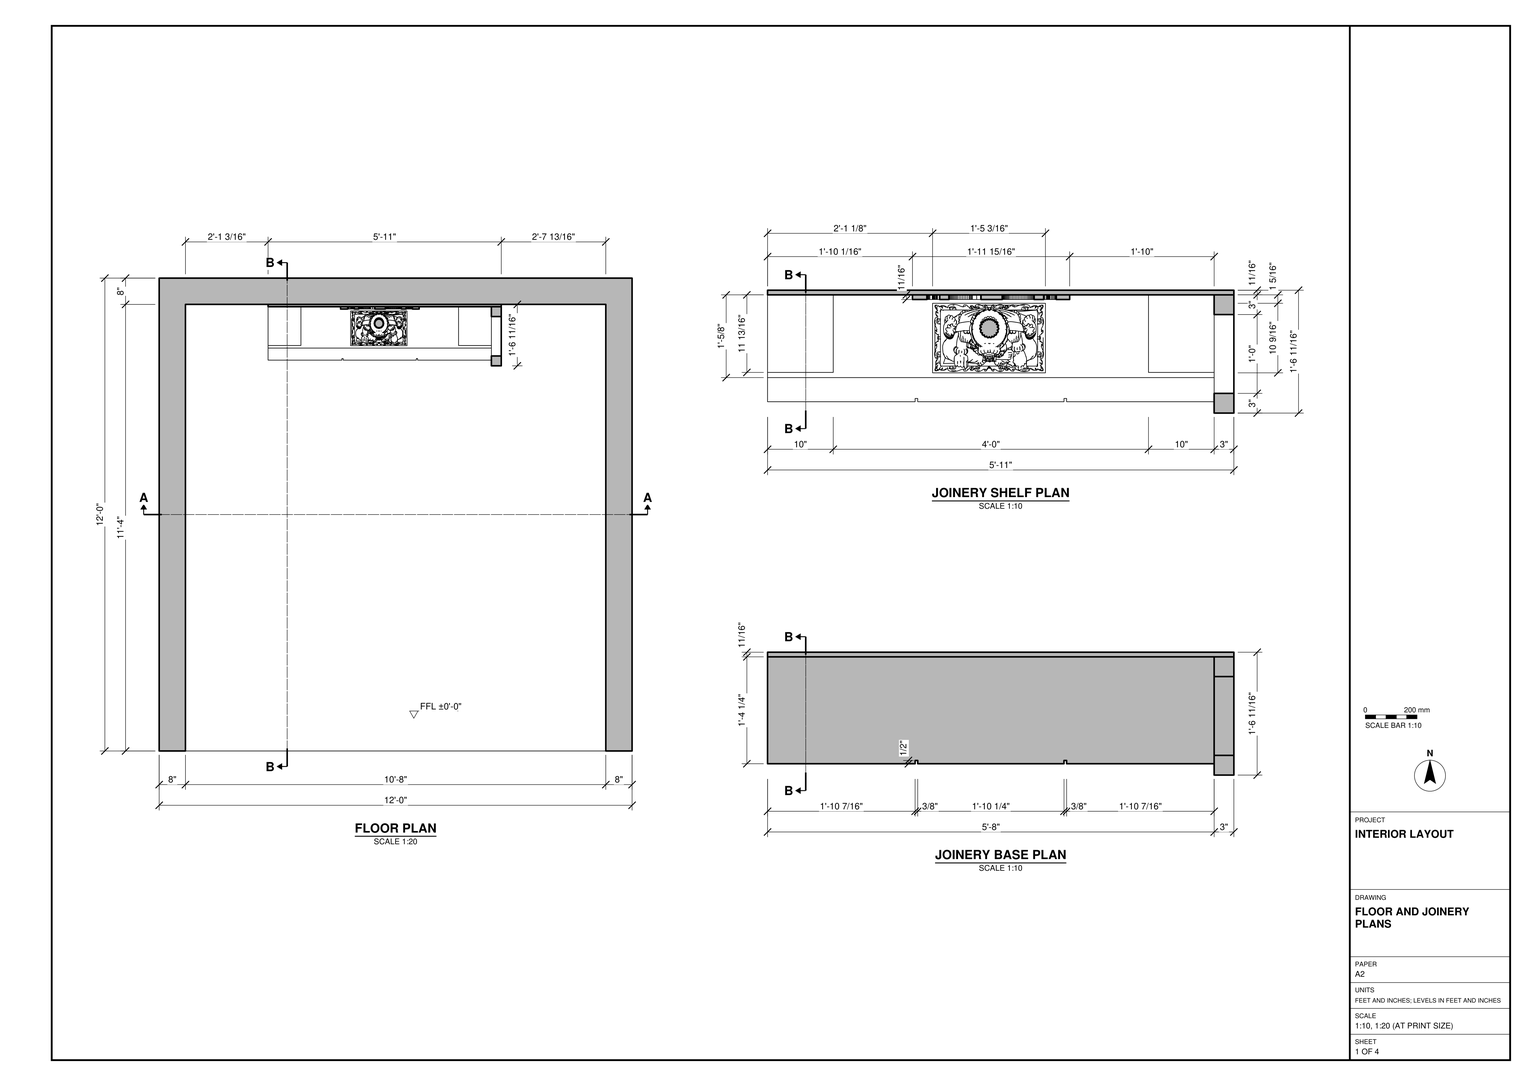
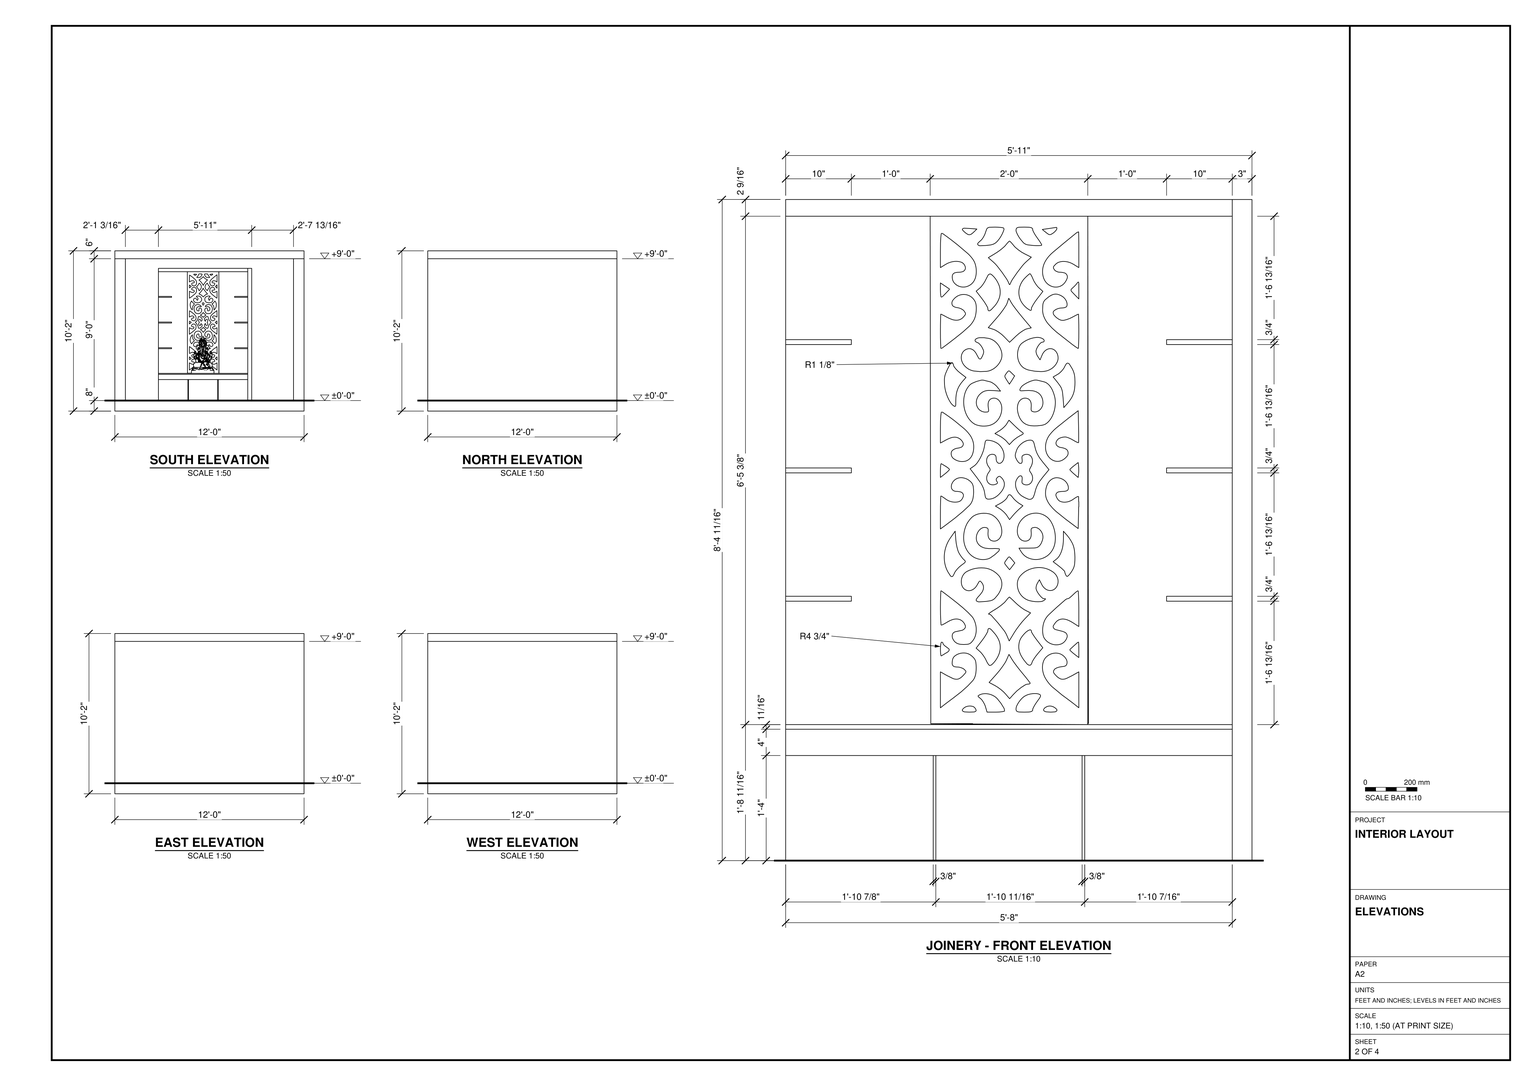
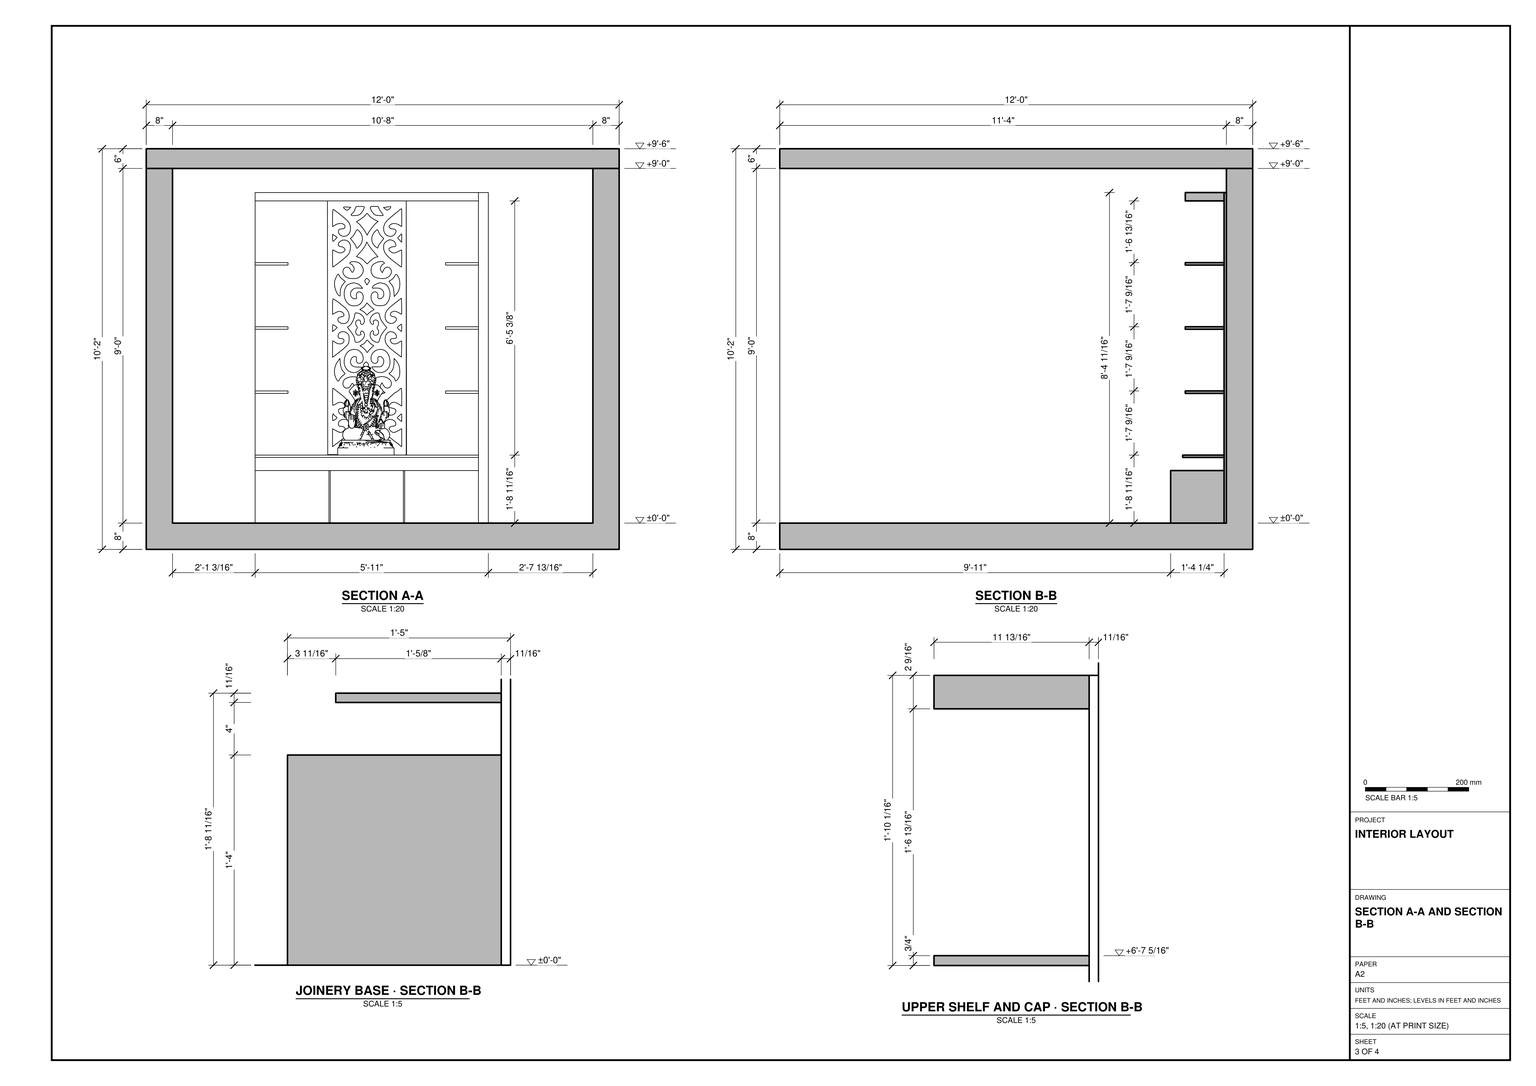
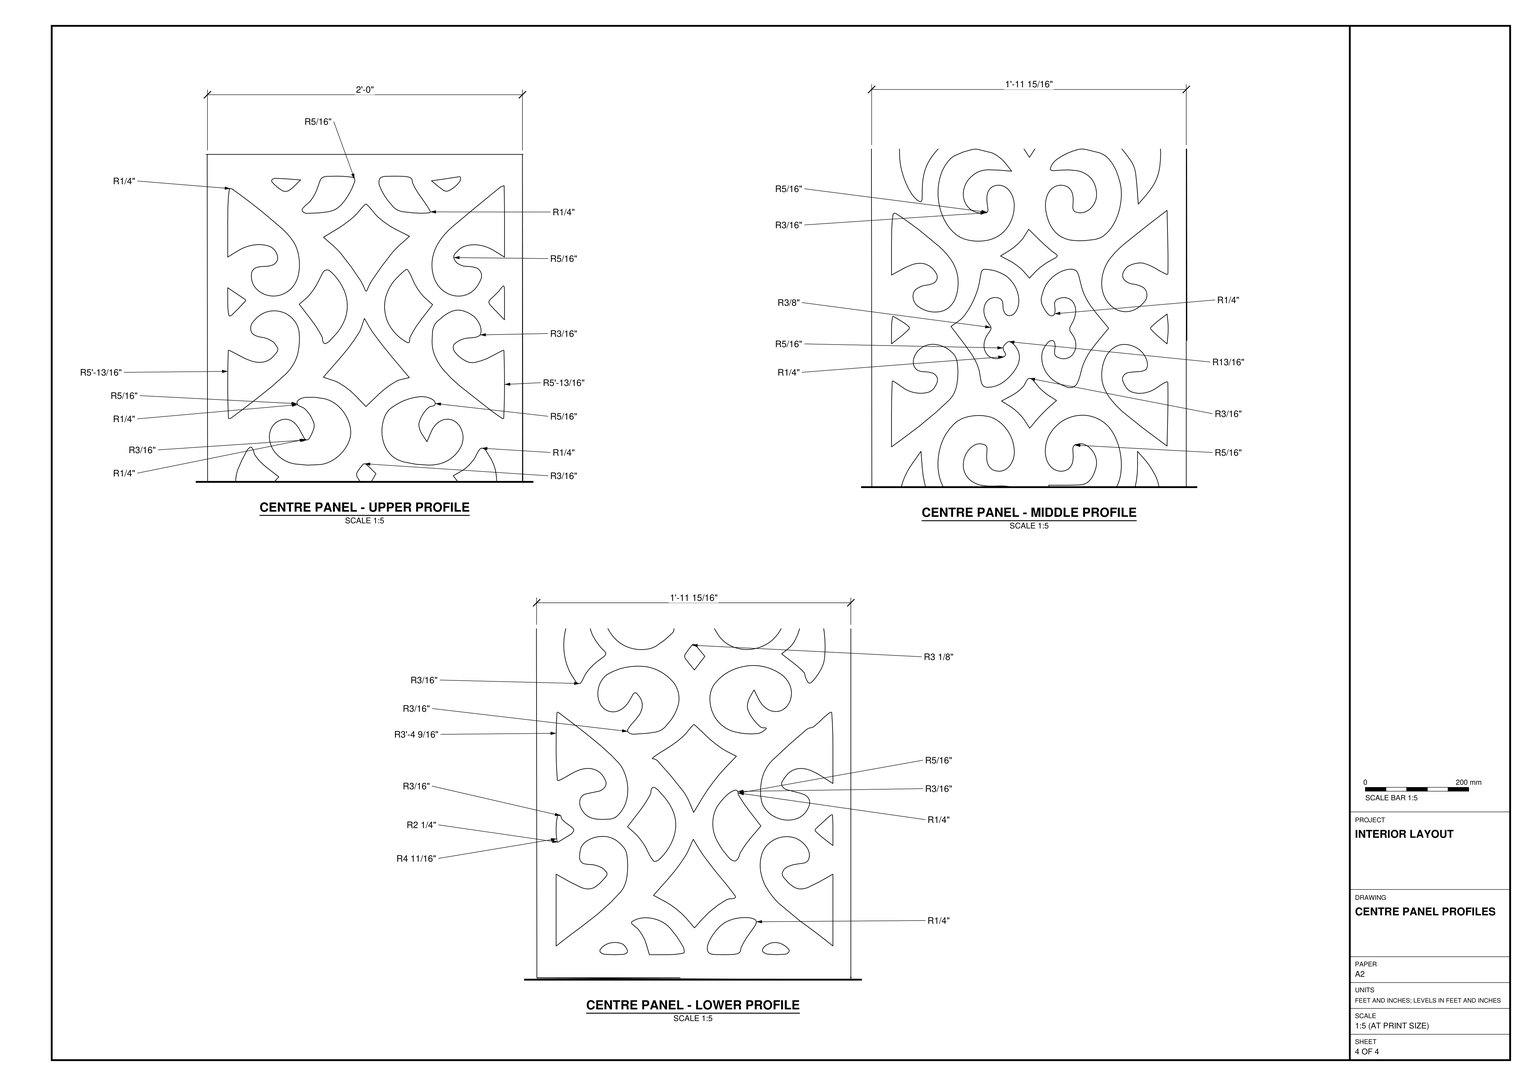
Build the room and its display unit in SketchUp using task_files/diagram_01.pdf. Work in feet and inches. The shell is 12'-0" wide by 12'-0" deep and 10'-2" high overall. Set the finished floor at ±0'-0". Model the 8" floor slab, the 8" north, east and west walls, and the 6" roof slab with its underside at +9'-0". Leave the south side open as shown in the floor plan and south elevation.

Place the display unit against the north wall, with its left edge 2'-1 3/16" from the inside face of the west wall. Build the low cabinet with three front divisions and leave a gap between its top and the display shelf above it. Use the joinery plans and sections to set the different projections of the cabinet, shelves, right end panel and top cap. Model the patterned cutouts in the central upright panel and align the short shelves in pairs on either side. Place a decorative figure on the display shelf in front of the patterned panel. Decor and loose items may be any suitable library components.

Keep the walls, floor slab, roof slab and built-in unit in separate groups or components, and use components for repeated parts such as matching shelves. Save one SketchUp model as output_files/open_front_room_with_built_in_display_joinery.skp.

# SketchUp Ruby script. Lengths in inches.
U = 1.inch
M = Sketchup.active_model
def pt(a) = Geom::Point3d.new(a.map { |v| v * U })
def face(e, loops, mat)
  f = e.add_face(loops[0].map { |a| pt(a) })
  loops[1..].each { |l| e.add_face(l.map { |a| pt(a) }).erase! }
  f.material = f.back_material = mat if mat
  f
end
# faces: each face lists its corners as indices into pts; further lists are holes
def faces(e, pts, list, mat = nil) = list.each { |f| face(e, (f[0].is_a?(Array) ? f : [f]).map { |l| l.map { |i| pts[i] } }, mat) }
# xy, xz, yz: faces in a plane at the given z, y or x. An outline is a flat list of corners, or four numbers for a rectangle; further outlines are holes
def ring(l) = l.size == 4 ? [[l[0], l[1]], [l[2], l[1]], [l[2], l[3]], [l[0], l[3]]] : l.each_slice(2).to_a
def flat(e, list, mat, &to3) = list.each { |f| face(e, (f[0].is_a?(Array) ? f : [f]).map { |l| ring(l).map { |u, v| to3.(u, v) } }, mat) }
def xy(e, z, list, mat = nil) = flat(e, list, mat) { |x, y| [x, y, z] }
def xz(e, y, list, mat = nil) = flat(e, list, mat) { |x, z| [x, y, z] }
def yz(e, x, list, mat = nil) = flat(e, list, mat) { |y, z| [x, y, z] }
def lines(e, pts, list) = list.each { |a, b| e.add_line(pt(pts[a]), pt(pts[b])) }
# prism: a flat outline (further loops are holes) pulled along v
def prism(e, loops, v, mat = nil)
  f = face(e, loops, mat); d = Geom::Vector3d.new(v.map { |x| x * U })
  f.pushpull(f.normal.samedirection?(d) ? d.length : -d.length)
end
def box(e, o, s, mat = nil) = prism(e, [[o, [o[0] + s[0], o[1], o[2]], [o[0] + s[0], o[1] + s[1], o[2]], [o[0], o[1] + s[1], o[2]]]], [0, 0, s[2]], mat)
def at(x, y, z, deg = 0) = Geom::Transformation.translation(pt([x, y, z])) * Geom::Transformation.rotation(ORIGIN, Z_AXIS, deg.degrees)
def axes(o, x, y, z) = Geom::Transformation.new([*x, 0, *y, 0, *z, 0, *pt(o).to_a, 1])
def part(name) = M.definitions.add(name)
# library, detail: a bought-in or finely detailed component or shape, given as its bounding box
def library(name, o, s) = part(name).tap { |d| box(d.entities, o, s) }
def detail(e, o, s) = box(e.add_group.entities, o, s)
def put(e, d, t, mat = nil) = e.add_instance(d, t).tap { |i| i.material = mat if mat }
def group(e, t, mat = nil) = e.add_group.tap { |g| g.transformation = t; g.material = mat if mat }.entities
root = M.entities
M.materials.add("[Color C04]").color = [255, 153, 50]
M.materials.add("[Color M00]").color = [255, 255, 255]
M.materials.add("[Color M03]").color = [170, 170, 170]
M.materials.add("[Color_B10]").color = [204, 173, 163]
M.materials.add("[Square Glass Tile 04]").color = [221, 197, 122]
M.materials.add("[Tile Hexagon White]").color = [213, 206, 204]
M.materials.add("[Wood Bamboo]").color = [177, 105, 43]
M.materials.add("[Wood OSB]").color = [240, 195, 122]
c1 = library("Ganesha+-+An+Do+Giao",[8.43,-11.04,-0.14],[9.49,5.78,12.28])
c2 = library("Group\#10",[0,-0.71,0],[24.14,0.71,77.4])
box(root,[0,0,116],[144,144,6])
xy(root,8,[[33.16,135.29,104.16,136]])
xy(root,108.66,[[33.16,135.29,104.16,136]])
xz(root,135.29,[[[33.16,8,104.16,108.66],[55.26,28.85,55.16,106.1,79.16,106.13,79.26,28.88]]])
xz(root,135.29,[[55.26,28.85,79.26,28.88,79.16,106.13,55.16,106.1]],"[Color C04]")
xz(root,136,[[33.16,8,104.16,108.66]])
yz(root,33.16,[[135.29,8,136,108.66]])
yz(root,104.16,[[135.29,8,136,108.66]])
put(root,c1,axes([43.04,143.63,29.03],[1.81,0,0],[0,1.83163,0],[0,0,2.31]))
g1 = group(root,at(33.16,135.29,86.57),"[Wood Bamboo]")
box(g1,[0,-11.8125,0],[10,11.8125,0.75])
g2 = group(root,at(33.16,135.29,67.04),"[Wood Bamboo]")
box(g2,[0,-11.8125,0],[10,11.8125,0.75])
g3 = group(root,at(33.16,135.29,47.5),"[Wood Bamboo]")
box(g3,[0,-11.8125,0],[10,11.8125,0.75])
g4 = group(root,at(91.16,135.29,47.5),"[Wood Bamboo]")
box(g4,[0,-11.8125,0],[10,11.8125,0.75])
g5 = group(root,at(91.16,135.29,67.04),"[Wood Bamboo]")
box(g5,[0,-11.8125,0],[10,11.8125,0.75])
g6 = group(root,at(91.16,135.29,86.57),"[Wood Bamboo]")
box(g6,[0,-11.8125,0],[10,11.8125,0.75])
g7 = group(root,at(33.16,135.29,8),"[Wood Bamboo]")
box(g7,[0,-11.8125,98.11],[68,11.8125,2.55])
g8 = group(root,at(33.16,135.29,8),"[Color_B10]")
prism(g8,[[[0,0,0],[68,0,0],[68,-16.27,0],[45.53,-16.27,0],[45.53,-15.77,0],[45.13,-15.77,0],[45.13,-16.27,0],[22.87,-16.27,0],[22.87,-15.77,0],[22.47,-15.77,0],[22.47,-16.27,0],[0,-16.27,0]]],[0,0,16])
box(g8,[0,-12.6,20],[68,12.6,0.71],"[Wood OSB]")
g9 = group(root,at(104.16,135.29,8,-90))
xy(g9,0,[[0,-3.01,18,0]],"[Wood Bamboo]")
xy(g9,3,[[3,-3.01,15,0]],"[Wood Bamboo]")
xy(g9,97.66,[[3,-3.01,15,0]],"[Wood Bamboo]")
xy(g9,100.66,[[0,-3.01,18,0]],"[Wood Bamboo]")
xz(g9,-3.01,[[[0,0,18,100.66],[3,3,15,97.66]]],"[Wood Bamboo]")
xz(g9,0,[[3,3,15,97.66]])
xz(g9,0,[[[0,0,18,100.66],[3,3,15,97.66]]],"[Wood Bamboo]")
yz(g9,0,[[-3.01,0,0,100.66]],"[Wood Bamboo]")
yz(g9,3,[[-3.01,3,0,97.66]],"[Wood Bamboo]")
yz(g9,15,[[-3.01,3,0,97.66]],"[Wood Bamboo]")
yz(g9,18,[[-3.01,0,0,100.66]],"[Wood Bamboo]")
put(root,c2,axes([55.16,135.29,28.71],[0.99425,0,0],[0,1,0],[0,0,1]),"[Color M03]")
g10 = group(root,at(0,0,0))
xy(g10,0,[[0,0,144,144]])
xy(g10,8,[[8,0,136,136]],"[Square Glass Tile 04]")
xy(g10,116,[[0,0,8,0,8,136,136,136,136,0,144,0,144,144,0,144]])
xz(g10,0,[[0,0,144,0,144,116,136,116,136,8,8,8,8,116,0,116]])
xz(g10,136,[[8,8,136,116]],"[Color M00]")
xz(g10,144,[[0,0,144,116]])
yz(g10,0,[[0,0,144,116]])
yz(g10,8,[[0,8,136,116]],"[Tile Hexagon White]")
yz(g10,136,[[0,8,136,116]],"[Tile Hexagon White]")
yz(g10,144,[[0,0,144,116]])
